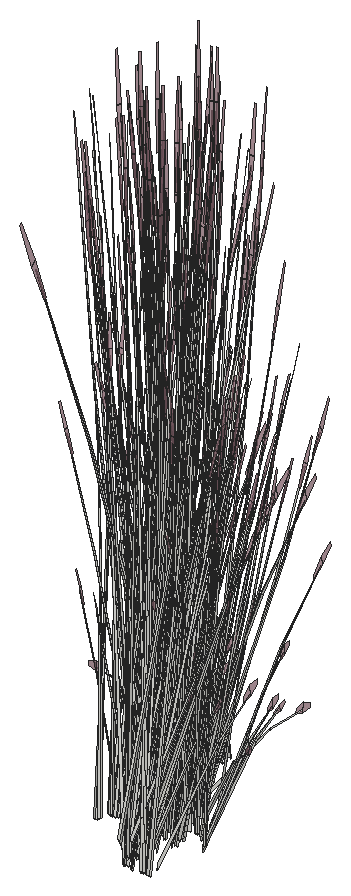
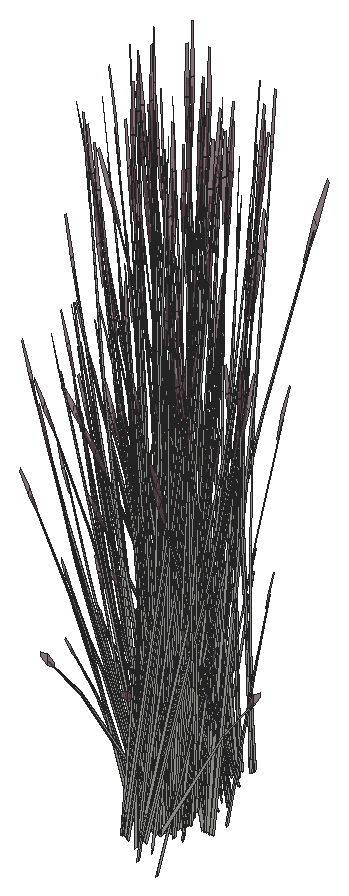
# SketchUp Ruby script. Lengths in inches.
U = 1.inch
M = Sketchup.active_model
def pt(a) = Geom::Point3d.new(a.map { |v| v * U })
def face(e, loops, mat)
  f = e.add_face(loops[0].map { |a| pt(a) })
  loops[1..].each { |l| e.add_face(l.map { |a| pt(a) }).erase! }
  f.material = f.back_material = mat if mat
  f
end
# faces: each face lists its corners as indices into pts; further lists are holes
def faces(e, pts, list, mat = nil) = list.each { |f| face(e, (f[0].is_a?(Array) ? f : [f]).map { |l| l.map { |i| pts[i] } }, mat) }
# xy, xz, yz: faces in a plane at the given z, y or x. An outline is a flat list of corners, or four numbers for a rectangle; further outlines are holes
def ring(l) = l.size == 4 ? [[l[0], l[1]], [l[2], l[1]], [l[2], l[3]], [l[0], l[3]]] : l.each_slice(2).to_a
def flat(e, list, mat, &to3) = list.each { |f| face(e, (f[0].is_a?(Array) ? f : [f]).map { |l| ring(l).map { |u, v| to3.(u, v) } }, mat) }
def xy(e, z, list, mat = nil) = flat(e, list, mat) { |x, y| [x, y, z] }
def xz(e, y, list, mat = nil) = flat(e, list, mat) { |x, z| [x, y, z] }
def yz(e, x, list, mat = nil) = flat(e, list, mat) { |y, z| [x, y, z] }
def lines(e, pts, list) = list.each { |a, b| e.add_line(pt(pts[a]), pt(pts[b])) }
# prism: a flat outline (further loops are holes) pulled along v
def prism(e, loops, v, mat = nil)
  f = face(e, loops, mat); d = Geom::Vector3d.new(v.map { |x| x * U })
  f.pushpull(f.normal.samedirection?(d) ? d.length : -d.length)
end
def box(e, o, s, mat = nil) = prism(e, [[o, [o[0] + s[0], o[1], o[2]], [o[0] + s[0], o[1] + s[1], o[2]], [o[0], o[1] + s[1], o[2]]]], [0, 0, s[2]], mat)
def at(x, y, z, deg = 0) = Geom::Transformation.translation(pt([x, y, z])) * Geom::Transformation.rotation(ORIGIN, Z_AXIS, deg.degrees)
def axes(o, x, y, z) = Geom::Transformation.new([*x, 0, *y, 0, *z, 0, *pt(o).to_a, 1])
def part(name) = M.definitions.add(name)
# library, detail: a bought-in or finely detailed component or shape, given as its bounding box
def library(name, o, s) = part(name).tap { |d| box(d.entities, o, s) }
def detail(e, o, s) = box(e.add_group.entities, o, s)
def put(e, d, t, mat = nil) = e.add_instance(d, t).tap { |i| i.material = mat if mat }
def group(e, t, mat = nil) = e.add_group.tap { |g| g.transformation = t; g.material = mat if mat }.entities
root = M.entities
M.materials.add("LightPink_Translucent").color = [144, 107, 117]
M.materials["LightPink_Translucent"].alpha = 0.75
c1 = part("blade")
p = [[2.15,0.21,22],[0,0.17,0],[0.09,0.45,0],[2.18,0.31,22],[2.29,0.31,22],[0.38,0.45,0],
  [2.48,0.24,33],[2.49,0.24,33],[2.48,0.22,33]]
faces(c1.entities,p,[[0,1,2,3],[4,5,2,3],[6,3,4,7],[8,0,3,6]])
c2 = part("seeds")
p = [[0.3,-0.1,1.38],[-0.01,-0.03,1.59],[-0.01,-0.03,0.03],[0.14,-0.07,-0.07],[0.29,-0.03,3],[0.15,0.01,3.11]]
faces(c2.entities,p,[[0,1,2,3],[1,0,4,5]],"LightPink_Translucent")
c3 = part("blade with seeds")
put(c3.entities,c1,at(0,0,0))
put(c3.entities,c2,axes([2.4,0.25,30.99],[1.5799,-0.05474,1.17369],[-0.12525,1.92788,0.29478],[-0.07173,-0.02425,1.56792]))
put(root,c3,axes([409.92,309.07,-10.02],[-0.35341,0.31182,-0.03625],[-0.32382,-0.34152,-0.16435],[-0.0228,-0.09677,0.54209]))
put(root,c3,axes([412.33,311.125,-7.3125],[-0.47307,-0.29971,-0.11324],[0.27254,-0.43404,-0.62851],[0.13365,-0.15087,0.95501]))
put(root,c3,axes([412.24,306.76,-7.36],[0.51122,0.01309,-0.66157],[-0.03434,0.5511,0.07984],[0.21658,0.05816,0.93586]))
put(root,c3,axes([411.67,307.21,-9.69],[0.47863,-0.27177,0.46235],[0.28609,0.48733,0],[-0.10901,0.0619,1.46668]))
put(root,c3,axes([410.37,312.76,-8.9],[0.44194,0.21918,1.40854],[-0.43295,0.47219,0.557],[-0.19393,-0.27986,1.18082]))
put(root,c3,axes([410.99,306.78,-9.87],[0.22235,0.62444,-0.05599],[-0.63531,0.21881,0],[0.00776,0.02181,1.60327]))
put(root,c3,axes([411.23,307.45,-10.11],[-0.47712,-0.13449,-0.28847],[0.12013,-0.47362,0.28847],[-0.09619,0.05462,1.29413]))
put(root,c3,axes([409.44,309.8,-7.3],[0.07899,0.43781,0.32977],[-0.45153,0.11561,-0.42575],[-0.12128,-0.12546,0.81462]))
put(root,c3,axes([408.0625,311.25,-10.12],[0,-0.54355,-0.46235],[0.57217,0,0],[0,-0.1238,1.46668]))
put(root,c3,axes([409.65,309.64,-10.12],[0.47863,-0.27177,-0.46235],[0.28609,0.48733,0],[0.10901,-0.0619,1.46668]))
put(root,c3,axes([412.49,310.58,-9.59],[-0.1827,-0.0161,1.33163],[-0.18717,-0.43188,-0.28638],[0.22444,-0.12218,0.56934]))
put(root,c3,axes([408.59,306.12,-7.3],[0.44516,-0.07768,0.32977],[0.11755,0.44407,-0.42575],[-0.12757,0.11927,0.81462]))
put(root,c3,axes([413.49,311,-7.62],[-0.0668,-0.00413,1.65179],[-0.27738,-0.44233,-0.15608],[0.11139,-0.14544,0.29231]))
put(root,c3,axes([413.08,305.65,-9.79],[0.63949,0,0],[0,0.60749,-0.48057],[0,0.13836,1.52448]))
put(root,c3,axes([412.82,305.96,-9.95],[-0.63917,-0.00435,-0.04634],[0,-0.60749,0.46507],[-0.02009,0.13829,1.47457]))
put(root,c3,axes([411.44,305.43,-9.52],[0.57594,0.25935,-0.27094],[-0.27732,0.5474,-0.46562],[0.0181,0.1344,1.4872]))
put(root,c3,axes([410.22,310.75,-10.08],[0.34446,-0.40855,-0.58063],[0.42791,0.37046,-0.15239],[0.13803,-0.10191,1.28164]))
put(root,c3,axes([412.7,309.78,-9.42],[-0.17034,0.27669,1.06958],[-0.14642,-0.37174,0.78586],[0.14069,-0.09315,0.23558]))
put(root,c3,axes([412.55,306.99,-7.78],[0.29098,0.34031,-0.32977],[-0.33226,0.32215,0.42575],[0.16881,0.04902,0.81462]))
put(root,c3,axes([412.69,306.05,-10.11],[-0.35699,0.33913,-0.28847],[-0.35699,-0.33913,0.28847],[0,0.10923,1.29413]))
put(root,c3,axes([411.15,306.08,-9.52],[0.05959,0.62022,-0.27094],[-0.62068,0.0375,-0.46562],[-0.1093,0.08261,1.4872]))
put(root,c3,axes([412.4,307.12,-7.6],[-0.02575,0.41332,0.05988],[-0.38885,-0.01133,0.47138],[0.14895,0.04325,0.71878]))
put(root,c3,axes([411.38,305.84,-9.94],[-0.24813,0.48978,-0.41661],[-0.51557,-0.23571,0.2005],[0,0.1129,1.33761]))
put(root,c3,axes([412.4375,306.99,-7.59],[-0.37709,0.35815,0.447],[-0.32522,-0.38035,0.36857],[0.17692,0.06607,0.92496]))
put(root,c3,axes([412.46,310.82,-7.78],[0.44516,-0.07768,-0.32977],[0.11755,0.44407,0.42575],[0.12757,-0.11927,0.81462]))
put(root,c3,axes([409.62,311.47,-9.94],[0.24813,-0.48978,-0.41661],[0.51557,0.23571,0.2005],[0,-0.1129,1.33761]))
put(root,c3,axes([409.84,311.23,-9.52],[-0.05959,-0.62022,-0.27094],[0.62068,-0.0375,-0.46562],[0.1093,-0.08261,1.4872]))
put(root,c3,axes([408.31,311.26,-10.11],[0.35699,-0.33913,-0.28847],[0.35699,0.33913,0.28847],[0,-0.10923,1.29413]))
put(root,c3,axes([407.58,307.38,-6.74],[0.45129,0.14509,-0.06041],[-0.13882,0.44656,-0.27392],[-0.07381,0.0678,0.90349]))
put(root,c3,axes([410.78,306.55,-10.08],[-0.34446,0.40855,-0.58063],[-0.42791,-0.37046,-0.15239],[-0.13803,0.10191,1.28164]))
put(root,c3,axes([408.16,309.63,-10.02],[-0.14753,0.44383,-0.03625],[-0.45406,-0.13653,-0.16435],[-0.06894,-0.07259,0.54209]))
put(root,c3,axes([412.09,311.09,-7.3],[-0.44516,0.07768,0.32977],[-0.11755,-0.44407,-0.42575],[0.12757,-0.11927,0.81462]))
put(root,c3,axes([409.56,311.875,-9.52],[-0.57594,-0.25935,-0.27094],[0.27732,-0.5474,-0.46562],[-0.0181,-0.1344,1.4872]))
put(root,c3,axes([411.24,307.41,-7.3],[-0.07899,-0.43781,0.32977],[0.45153,-0.11561,-0.42575],[0.12128,0.12546,0.81462]))
put(root,c3,axes([407.92,311.66,-9.79],[-0.63949,0,0],[0,-0.60749,-0.48057],[0,-0.13836,1.52448]))
put(root,c3,axes([411.39,307.24,-9.83],[0.64025,0.17667,0.2864],[-0.16018,0.63149,-0.33981],[-0.10597,0.07904,1.53541]))
put(root,c3,axes([411.35,307.67,-10.12],[-0.47863,0.27177,-0.46235],[-0.28609,-0.48733,0],[-0.10901,0.0619,1.46668]))
put(root,c3,axes([412.9375,306.06,-10.12],[0,0.54355,-0.46235],[-0.57217,0,0],[0,0.1238,1.46668]))
put(root,c3,axes([411.51,306.12,-8.39],[-0.18996,-0.09365,1.59586],[0.39312,-0.39287,0.12904],[0.24502,0.17723,0.68222]))
put(root,c3,axes([409.76,309.85,-10.11],[0.47712,0.13449,-0.28847],[-0.12013,0.47362,0.28847],[0.09619,-0.05462,1.29413]))
put(root,c3,axes([411.54,304.89,-7.83],[-0.44191,-0.28242,1.28769],[0.46662,-0.43971,0.5556],[0.14258,0.26499,1.24467]))
put(root,c3,axes([408.36,306.08,-7.3125],[0.47307,0.29971,-0.11324],[-0.27254,0.43404,-0.62851],[-0.13365,0.15087,0.95501]))
put(root,c3,axes([412.21,307.1875,-9.42],[-0.28795,-0.15629,1.06958],[0.37181,-0.1588,0.78586],[0.10029,0.13452,0.23558]))
put(root,c3,axes([411.2,307.63,-7.3125],[0.30474,-0.46525,-0.11324],[0.44133,0.26804,-0.62851],[0.15341,0.13145,0.95501]))
put(root,c3,axes([412.5,311.02,-7.6],[0.35109,0.22859,0.05988],[-0.2044,0.32553,0.47138],[0.11256,-0.10524,0.71878]))
put(root,c3,axes([412.4,310.92,-7.59],[0.12683,0.50025,0.447],[-0.49754,0.08682,0.36857],[0.14663,-0.11765,0.92496]))
put(root,c3,axes([413.74,311.53,-7.61],[0.07097,-0.08279,1.62908],[-0.09083,-0.50786,-0.25764],[0.17806,-0.09629,0.13065]))
put(root,c3,axes([409.1875,307,-7.3],[0.34603,-0.28618,0.32977],[0.32756,0.32677,-0.42575],[-0.04984,0.16603,0.81462]))
put(root,c3,axes([411.78,307.58,-9.79],[0.31974,0.54466,0],[-0.53494,0.30375,-0.48057],[-0.12184,0.06918,1.52448]))
put(root,c3,axes([408.41,311.5,-9.83],[-0.47569,0.45698,0.2864],[-0.47598,-0.45217,-0.33981],[-0.01661,-0.12977,1.53541]))
put(root,c3,axes([410.8,308.02,-7.62],[0.00151,-0.06581,1.65179],[0.43826,-0.29033,-0.15608],[0.15223,0.10363,0.29231]))
put(root,c3,axes([412.29,307.77,-10.61],[0.03726,-0.07847,1.6421],[0.46909,-0.23111,-0.25086],[0.14221,0.11962,0.2797]))
put(root,c3,axes([411.51,305.43,-9.35],[-0.01397,-0.51177,1.31553],[0.63227,0.13266,0.557],[-0.14954,0.28003,1.24175]))
put(root,c3,axes([411.67,305.98,-10.05],[0.18752,0.49766,-0.6445],[-0.54017,0.17923,-0.16915],[0.02073,0.16852,1.42262]))
put(root,c3,axes([408.875,307.26,-7.6],[-0.42027,-0.02533,0.05988],[0.01152,-0.38243,0.47138],[-0.04398,0.14649,0.71878]))
put(root,c3,axes([409.01,307.3,-7.59],[-0.36417,-0.37086,0.447],[0.38674,-0.31985,0.36857],[-0.06718,0.174,0.92496]))
put(root,c3,axes([411.56,307.4,-7.64],[0.50465,-0.12921,-0.47583],[0.08828,0.48932,-0.36857],[0.13555,0.14022,0.91046]))
put(root,c3,axes([409.93,311.71,-9.73],[0.57623,0.26344,0.22409],[-0.27732,0.5474,0.46562],[0,-0.12618,1.49497]))
put(root,c3,axes([409.7,312.45,-9.73],[0.13555,-0.64407,-0.21817],[0.64269,0.11227,0.47743],[-0.1123,-0.08895,1.45677]))
put(root,c3,axes([410.16,307.47,-7.3],[0.15418,-0.41799,0.32977],[0.44981,0.12192,-0.42575],[0.04124,0.16829,0.81462]))
put(root,c3,axes([412.26,307.9,-9.52],[-0.32795,-0.01705,0.97832],[0.21658,-0.36206,0.54015],[0.12956,0.12863,0.76741]))
put(root,c3,axes([409.74,311.35,-9.47],[-0.55535,0.03355,0.41661],[-0.05022,-0.55698,-0.2005],[0.09942,-0.05645,1.33761]))
put(root,c3,axes([411.3125,307.8,-7.6],[-0.23243,0.34529,0.05988],[-0.331,-0.20103,0.47138],[0.10701,0.1107,0.71878]))
put(root,c3,axes([408.31,311.75,-9.69],[0,0.54355,0.46235],[-0.57217,0,0],[0,-0.1238,1.46668]))
put(root,c3,axes([410.76,308.97,-6.74],[0.35341,-0.31182,-0.06041],[0.32382,0.34152,-0.27392],[0.0228,0.09677,0.90349]))
put(root,c3,axes([412.34,312.3,-7.3125],[-0.25732,-0.49218,-0.11324],[0.45669,-0.24187,-0.62851],[0.19245,-0.06494,0.95501]))
put(root,c3,axes([412.32,311.875,-7.64],[0.13855,-0.49442,-0.47583],[0.47502,0.16947,-0.36857],[0.19125,-0.04534,0.91046]))
put(root,c3,axes([411.57,309.86,-9.79],[0.31974,-0.54466,0],[0.53494,0.30375,-0.48057],[0.12184,0.06918,1.52448]))
put(root,c3,axes([411.41,307.71,-7.59],[-0.50866,0.12474,0.447],[-0.08828,-0.48932,0.36857],[0.11963,0.14421,0.92496]))
put(root,c3,axes([409.66,312.19,-9.94],[-0.30722,-0.45622,-0.41661],[0.46535,-0.32126,0.2005],[-0.09942,-0.05645,1.33761]))
put(root,c3,axes([409.72,311.55,-9.8],[0.22235,0.6078,0.42607],[-0.63531,0.21135,0.16719],[0.00776,-0.11168,1.47927]))
put(root,c3,axes([412.83,312.01,-10.15],[-0.32938,0.06523,1.31842],[-0.05243,-0.51922,0.07547],[0.2307,-0.07859,0.75023]))
put(root,c3,axes([413.43,311.55,-9.89],[-0.31706,-0.34757,-0.06041],[0.34725,-0.31847,-0.27392],[0.09839,-0.02242,0.90349]))
put(root,c3,axes([411.18,307.02,-9.59],[0.00902,-0.18018,1.33163],[0.43127,-0.20126,-0.28638],[0.13313,0.21566,0.56934]))
put(root,c3,axes([409.61,312.03,-9.47],[-0.24813,0.48978,0.41661],[-0.51557,-0.23571,-0.2005],[0,-0.1129,1.33761]))
put(root,c3,axes([410.52,311.6,-9.95],[0,-0.62892,0],[0.63949,0,0],[0,0,1.6711]))
put(root,c3,axes([410.02,307.85,-7.6],[-0.37684,0.18473,0.05988],[-0.18445,-0.33686,0.47138],[0.03639,0.14849,0.71878]))
put(root,c3,axes([409.01,307.41,-7.78],[-0.34603,0.28618,-0.32977],[-0.32756,-0.32677,0.42575],[-0.04984,0.16603,0.81462]))
put(root,c3,axes([411.3,310.15,-9.69],[-0.47863,-0.27177,0.46235],[0.28609,-0.48733,0],[0.10901,0.0619,1.46668]))
put(root,c3,axes([408.97,307.08,-6.97],[0.56206,0.02693,-0.12569],[-0.01536,0.50991,-0.69765],[-0.03904,0.19638,1.06006]))
put(root,c3,axes([412.23,312.05,-7.36],[0.44939,-0.24006,-0.66157],[0.25044,0.49415,0.07984],[0.21713,-0.05613,0.93586]))
put(root,c3,axes([410.01,307.65,-7.3125],[0.50045,-0.25306,-0.11324],[0.24593,0.44915,-0.62851],[0.06603,0.18927,0.95501]))
put(root,c3,axes([410.15,307.82,-7.28],[-0.50393,-0.1421,0.49617],[0.17232,-0.46717,0.40911],[0.03028,0.18372,1.0267]))
put(root,c3,axes([409.23,308.52,-9.42],[-0.01324,-0.32319,1.06958],[0.33072,0.23052,0.78586],[-0.06504,0.15405,0.23558]))
put(root,c3,axes([410.22,311.2,-9.8],[-0.42403,0.49328,0.42607],[-0.50377,-0.43543,0.16719],[0.10223,-0.04923,1.47927]))
put(root,c3,axes([410.68,312.09,-9.86],[-0.47569,-0.46784,-0.05709],[0.47598,-0.46812,0],[-0.01661,-0.01634,1.63492]))
put(root,c3,axes([410.1,307.75,-10.61],[0.08277,-0.02958,1.6421],[0.49786,0.16279,-0.25086],[0.01456,0.18348,0.2797]))
put(root,c3,axes([409.48,310.39,-9.7],[-0.14774,0.54019,0.16428],[-0.54062,-0.15287,0.32672],[0.09339,-0.00263,1.49371]))
put(root,c3,axes([412.17,312.15,-7.3],[-0.42502,-0.15163,0.32977],[0.12396,-0.44238,-0.42575],[0.17112,-0.04056,0.81462]))
put(root,c3,axes([409.26,310.83,-10.52],[-0.50338,0.21762,1.20058],[-0.16022,-0.62439,0.4665],[0.30911,0.01039,1.36553]))
put(root,c3,axes([410.61,310.99,-9.5625],[0.09866,-0.48509,0.13483],[0.48202,0.0842,-0.38503],[0.08772,0.04981,1.18024]))
put(root,c3,axes([409.35,307.27,-7.34],[0.3661,0.36521,-0.52818],[-0.38674,0.31985,-0.40911],[-0.0557,0.18556,1.01061]))
put(root,c3,axes([409.78,312.14,-9.8],[0.64638,0.11452,0.42607],[-0.13155,0.64678,0.16719],[-0.09446,-0.06245,1.47927]))
put(root,c3,axes([408.96,307.82,-9.37],[0.46459,-0.09625,0.0606],[0.10681,0.38778,-0.80367],[-0.02945,0.1963,0.72038]))
put(root,c3,axes([410.4375,307.63,-7.64],[0.50273,0.13626,-0.47583],[-0.17232,0.46717,-0.36857],[0.0461,0.18809,0.91046]))
put(root,c3,axes([413.1875,311.67,-10.61],[-0.02673,-0.08252,1.6421],[0.18538,-0.48271,-0.25086],[0.187,-0.00694,0.2797]))
put(root,c3,axes([410.72,306.66,-8.39],[-0.1169,-0.17452,1.59586],[0.54019,-0.14692,0.12904],[0.12209,0.27397,0.68222]))
put(root,c3,axes([410.4,311.12,-9.47],[-0.30722,-0.45622,0.41661],[0.46535,-0.32126,-0.2005],[0.09942,0.05645,1.33761]))
put(root,c3,axes([408.82,313.2,-10.11],[-0.12013,-0.47362,-0.28847],[0.47712,-0.13449,0.28847],[-0.09619,-0.05462,1.29413]))
put(root,c3,axes([410.21,307.92,-7.78],[-0.15418,0.41799,-0.32977],[-0.44981,-0.12192,0.42575],[0.04124,0.16829,0.81462]))
put(root,c3,axes([409.43,313.18,-9.7],[0.54955,-0.14427,0.16428],[0.1357,0.53689,0.32672],[-0.04901,-0.07823,1.49371]))
put(root,c3,axes([410.5625,311.15,-9.52],[0.51635,-0.36087,-0.27094],[0.34336,0.5099,-0.46562],[0.1274,0.05178,1.4872]))
put(root,c3,axes([412.61,312.1,-7.78],[0.42502,0.15163,-0.32977],[-0.12396,0.44238,0.42575],[0.17112,-0.04056,0.81462]))
put(root,c3,axes([409.24,307.11,-7.03],[-0.01331,0.50278,-0.73435],[-0.56035,-0.03377,0.08862],[-0.05914,0.213,1.03881]))
put(root,c3,axes([407.77,308.43,-7.62],[0.05802,-0.03282,1.65179],[0.47954,0.21828,-0.15608],[-0.01127,0.18175,0.29231]))
put(root,c3,axes([411.86,310.1875,-10.12],[0.47863,0.27177,-0.46235],[-0.28609,0.48733,0],[0.10901,0.0619,1.46668]))
put(root,c3,axes([410.95,311.74,-9.95],[0.57217,0,0],[0,0.56272,0],[0,0,1.66132]))
put(root,c3,axes([409.77,306.75,-8.39],[-0.01252,-0.20862,1.59586],[0.54251,0.1384,0.12904],[-0.03356,0.2973,0.68222]))
put(root,c3,axes([409.98,312.45,-9.52],[-0.51635,0.36087,-0.27094],[-0.34336,-0.5099,-0.46562],[-0.1274,-0.05178,1.4872]))
put(root,c3,axes([411.12,310.42,-9.7],[-0.54955,0.14427,0.16428],[-0.1357,-0.53689,0.32672],[0.04901,0.07823,1.49371]))
put(root,c3,axes([411.46,311.55,-8.39],[-0.21212,0.01231,1.59586],[0.14072,-0.53355,0.12904],[0.3023,0.033,0.68222]))
put(root,c3,axes([411.73,310.39,-10.11],[0.12013,0.47362,-0.28847],[-0.47712,0.13449,0.28847],[0.09619,0.05462,1.29413]))
put(root,c3,axes([410.26,307.54,-7.36],[0.24409,0.44196,-0.66157],[-0.50245,0.2463,0.07984],[0.05708,0.21354,0.93586]))
put(root,c3,axes([412.55,312.29,-7.6],[0.18783,0.37061,0.05988],[-0.34252,0.1814,0.47138],[0.15099,-0.03579,0.71878]))
put(root,c3,axes([408.84,308.23,-9.59],[0.16138,-0.08575,1.33163],[0.39845,0.25854,-0.28638],[-0.1186,0.22371,0.56934]))
put(root,c3,axes([410.77,311.45,-9.78],[-0.64638,-0.11452,0.45814],[0.13155,-0.64678,0.17978],[0.09446,0.06245,1.59061]))
put(root,c3,axes([409.89,308.66,-7.61],[0.06483,0.08753,1.62908],[0.52315,0.03439,-0.25764],[0.05261,0.19303,0.13065]))
put(root,c3,axes([412.51,312.15,-7.59],[-0.14449,0.4956,0.447],[-0.47502,-0.16947,0.36857],[0.1868,-0.02978,0.92496]))
put(root,c3,axes([410.25,313.05,-9.95],[-0.16686,-0.46861,0],[0.47648,-0.16411,0],[0,0,1.4375]))
put(root,c3,axes([409.94,312.6,-9.5625],[-0.09866,0.48509,0.13483],[-0.48202,-0.0842,-0.38503],[-0.08772,-0.04981,1.18024]))
put(root,c3,axes([410.88,312.98,-9.97],[0.53691,-0.18442,-0.17877],[0.18866,0.53125,0.00007],[0.05927,-0.02038,1.61933]))
put(root,c3,axes([411.0625,313.21,-9.7],[0.14774,-0.54019,0.16428],[0.54062,0.15287,0.32672],[-0.09339,0.00263,1.49371]))
put(root,c3,axes([410.94,311.98,-9.9375],[0.35699,0.35109,0],[-0.35699,0.35109,0],[0,0,1.57621]))
put(root,c3,axes([411.91,311.83,-9.7],[-0.40181,-0.39593,0.16428],[0.40492,-0.38402,0.32672],[-0.04438,0.08086,1.49371]))
put(root,c3,axes([411.16,311.23,-10.08],[0.53199,0.08911,-0.58063],[-0.11226,0.54969,-0.15239],[0.15876,0.06661,1.28164]))
put(root,c3,axes([413.51,312.1875,-9.42],[-0.31598,0.08973,1.06958],[0.14873,-0.37085,0.78586],[0.16763,0.02538,0.23558]))
put(root,c3,axes([410.14,313.26,-9.95],[-0.51557,-0.24403,0],[0.24813,-0.50705,0],[0,0,1.51513]))
put(root,c3,axes([410.5625,312.61,-9.7],[-0.49938,-0.43748,-0.23459],[0.42021,-0.49126,0.51337],[-0.13447,0.05118,1.56642]))
put(root,c3,axes([409.25,313.45,-9.69],[0.47863,0.27177,0.46235],[-0.28609,0.48733,0],[-0.10901,-0.0619,1.46668]))
put(root,c3,axes([409.05,307.82,-8.87],[0.01124,-0.2806,1.43727],[0.50537,0.14821,0.19862],[-0.04379,0.29905,0.67868]))
put(root,c3,axes([410.9375,311.57,-9.47],[0.24813,-0.48978,0.41661],[0.51557,0.23571,-0.2005],[0,0.1129,1.33761]))
put(root,c3,axes([413.37,313.76,-7.62],[-0.04624,-0.04758,1.65179],[0.10116,-0.51007,-0.15608],[0.18215,-0.03259,0.29231]))
put(root,c3,axes([410.84,311.85,-9.87],[0,0.62861,-0.05249],[-0.63949,0,0],[0,0.01975,1.67027]))
put(root,c3,axes([410.89,311.4,-9.94],[0.30722,0.45622,-0.41661],[-0.46535,0.32126,0.2005],[0.09942,0.05645,1.33761]))
put(root,c3,axes([412.97,313.33,-8.34],[-0.09788,-0.45691,-0.03251],[0.46264,-0.10504,-0.14742],[0.09661,0.02897,0.48626]))
put(root,c3,axes([411.77,313.32,-7.3125],[0.02738,-0.55277,-0.11324],[0.51847,0.01511,-0.62851],[0.19968,0.0384,0.95501]))
put(root,c3,axes([412.24,311.84,-9.69],[0,-0.54355,0.46235],[0.57217,0,0],[0,0.1238,1.46668]))
put(root,c3,axes([410.81,312.25,-9.47],[0.55535,-0.03355,0.41661],[0.05022,0.55698,-0.2005],[-0.09942,0.05645,1.33761]))
put(root,c3,axes([411.15,311.68,-9.5625],[0.47648,-0.15851,0.13483],[0.16686,0.45265,-0.38503],[0,0.09962,1.18024]))
put(root,c3,axes([411.6875,313.1,-7.3],[-0.29098,-0.34031,0.32977],[0.33226,-0.32215,-0.42575],[0.16881,0.04902,0.81462]))
put(root,c3,axes([410.3125,312.52,-9.94],[-0.55535,0.03355,-0.41661],[-0.05022,-0.55698,0.2005],[-0.09942,0.05645,1.33761]))
put(root,c3,axes([407.97,316.9,-7.61],[-0.07822,-0.07621,1.62908],[-0.52201,0.04832,-0.25764],[-0.08331,-0.18228,0.13065]))
put(root,c3,axes([409.18,317.8,-9.59],[-0.14537,0.11002,1.33163],[-0.43536,-0.19256,-0.28638],[0.0807,-0.23948,0.56934]))
put(root,c3,axes([412.92,312.78,-9.59],[-0.12317,-0.13368,1.33163],[0.16025,-0.44223,-0.28638],[0.24919,0.05991,0.56934]))
put(root,c3,axes([408.52,318.18,-7.36],[-0.24409,-0.44196,-0.66157],[0.50245,-0.2463,0.07984],[-0.05708,-0.21354,0.93586]))
put(root,c3,axes([410.72,313.27,-9.95],[0.51557,0.24403,0],[-0.24813,0.50705,0],[0,0,1.62917]))
put(root,c3,axes([408.1,317.2,-10.61],[-0.08578,0.01958,1.6421],[-0.47437,-0.22044,-0.25086],[0.00796,-0.18387,0.2797]))
put(root,c3,axes([412.22,312.99,-7.61],[0.10971,-0.00919,1.62908],[0.30091,-0.42228,-0.25764],[0.19514,0.05574,0.13065]))
put(root,c3,axes([410.93,313.81,-9.96],[-0.31576,-0.54657,-0.04789],[0.53494,-0.30375,0.48057],[-0.13182,0.05204,1.52373]))
put(root,c3,axes([410.81,312.49,-9.5625],[0.37783,0.32657,0.13483],[-0.31516,0.36844,-0.38503],[-0.08772,0.04981,1.18024]))
put(root,c3,axes([409.54,318.62,-7.36],[0.01331,-0.50278,-0.66157],[0.56035,0.03377,0.07984],[0.05914,-0.213,0.93586]))
put(root,c3,axes([410.32,317.83,-7.61],[-0.00494,-0.10818,1.62908],[-0.41695,-0.31265,-0.25764],[0.06446,-0.18952,0.13065]))
put(root,c3,axes([408.57,317.81,-7.78],[0.15418,-0.41799,-0.32977],[0.44981,0.12192,0.42575],[-0.04124,-0.16829,0.81462]))
put(root,c3,axes([408.91,318.36,-8.39],[-0.09522,0.18683,1.59586],[-0.39947,-0.38663,0.12904],[0.18021,-0.24097,0.68222]))
put(root,c3,axes([410.21,317.44,-7.62],[-0.05194,0.04152,1.65179],[-0.50886,-0.14007,-0.15608],[-0.01842,-0.18118,0.29231]))
put(root,c3,axes([411.79,313.05,-7.36],[0.51122,0.01309,-0.66157],[-0.03434,0.5511,0.07984],[0.21658,0.05816,0.93586]))
put(root,c3,axes([411.22,313.49,-9.69],[0.47863,-0.27177,0.46235],[0.28609,0.48733,0],[-0.10901,0.0619,1.46668]))
put(root,c3,axes([408.34,318.09,-7.64],[-0.50273,-0.13626,-0.47583],[0.17232,-0.46717,-0.36857],[-0.0461,-0.18809,0.91046]))
put(root,c3,axes([410.54,313.07,-9.87],[0.22235,0.62444,-0.05599],[-0.63531,0.21881,0],[0.00776,0.02181,1.60327]))
put(root,c3,axes([408.65,316.92,-9.42],[0.06561,0.31695,1.06958],[-0.36394,-0.17555,0.78586],[0.03916,-0.16229,0.23558]))
put(root,c3,axes([410.78,313.74,-10.11],[-0.47712,-0.13449,-0.28847],[0.12013,-0.47362,0.28847],[-0.09619,0.05462,1.29413]))
put(root,c3,axes([409.42,318.45,-7.64],[-0.3661,-0.36521,-0.47583],[0.38674,-0.31985,-0.36857],[0.0557,-0.18556,0.91046]))
put(root,c3,axes([408.14,312.41,-7.3],[0.44516,-0.07768,0.32977],[0.11755,0.44407,-0.42575],[-0.12757,0.11927,0.81462]))
put(root,c3,axes([412.63,311.93,-9.79],[0.63949,0,0],[0,0.60749,-0.48057],[0,0.13836,1.52448]))
put(root,c3,axes([412.37,312.25,-9.95],[-0.63917,-0.00435,-0.04634],[0,-0.60749,0.46507],[-0.02009,0.13829,1.47457]))
put(root,c3,axes([410.99,311.72,-9.52],[0.57594,0.25935,-0.27094],[-0.27732,0.5474,-0.46562],[0.0181,0.1344,1.4872]))
put(root,c3,axes([412.1,313.28,-7.78],[0.29098,0.34031,-0.32977],[-0.33226,0.32215,0.42575],[0.16881,0.04902,0.81462]))
put(root,c3,axes([412.24,312.34,-10.11],[-0.35699,0.33913,-0.28847],[-0.35699,-0.33913,0.28847],[0,0.10923,1.29413]))
put(root,c3,axes([410.7,312.37,-9.52],[0.05959,0.62022,-0.27094],[-0.62068,0.0375,-0.46562],[-0.1093,0.08261,1.4872]))
put(root,c3,axes([411.95,313.41,-7.6],[-0.02575,0.41332,0.05988],[-0.38885,-0.01133,0.47138],[0.14895,0.04325,0.71878]))
put(root,c3,axes([410.93,312.125,-9.94],[-0.24813,0.48978,-0.41661],[-0.51557,-0.23571,0.2005],[0,0.1129,1.33761]))
put(root,c3,axes([408.625,317.9,-7.59],[0.50393,0.1421,0.447],[-0.17232,0.46717,0.36857],[-0.03028,-0.18372,0.92496]))
put(root,c3,axes([411.99,313.28,-7.59],[-0.37709,0.35815,0.447],[-0.32522,-0.38035,0.36857],[0.17692,0.06607,0.92496]))
put(root,c3,axes([408.77,318.07,-7.3125],[-0.50045,0.25306,-0.11324],[-0.24593,-0.44915,-0.62851],[-0.06603,-0.18927,0.95501]))
put(root,c3,axes([409.81,318.64,-7.3125],[-0.56206,-0.02693,-0.11324],[0.01536,-0.50991,-0.62851],[0.03904,-0.19638,0.95501]))
put(root,c3,axes([409.77,318.3125,-7.78],[0.34603,-0.28618,-0.32977],[0.32756,0.32677,0.42575],[0.04984,-0.16603,0.81462]))
put(root,c3,axes([408.76,317.87,-7.6],[0.37684,-0.18473,0.05988],[0.18445,0.33686,0.47138],[-0.03639,-0.14849,0.71878]))
put(root,c3,axes([407.125,313.67,-6.74],[0.45129,0.14509,-0.06041],[-0.13882,0.44656,-0.27392],[-0.07381,0.0678,0.90349]))
put(root,c3,axes([410.33,312.84,-10.08],[-0.34446,0.40855,-0.58063],[-0.42791,-0.37046,-0.15239],[-0.13803,0.10191,1.28164]))
